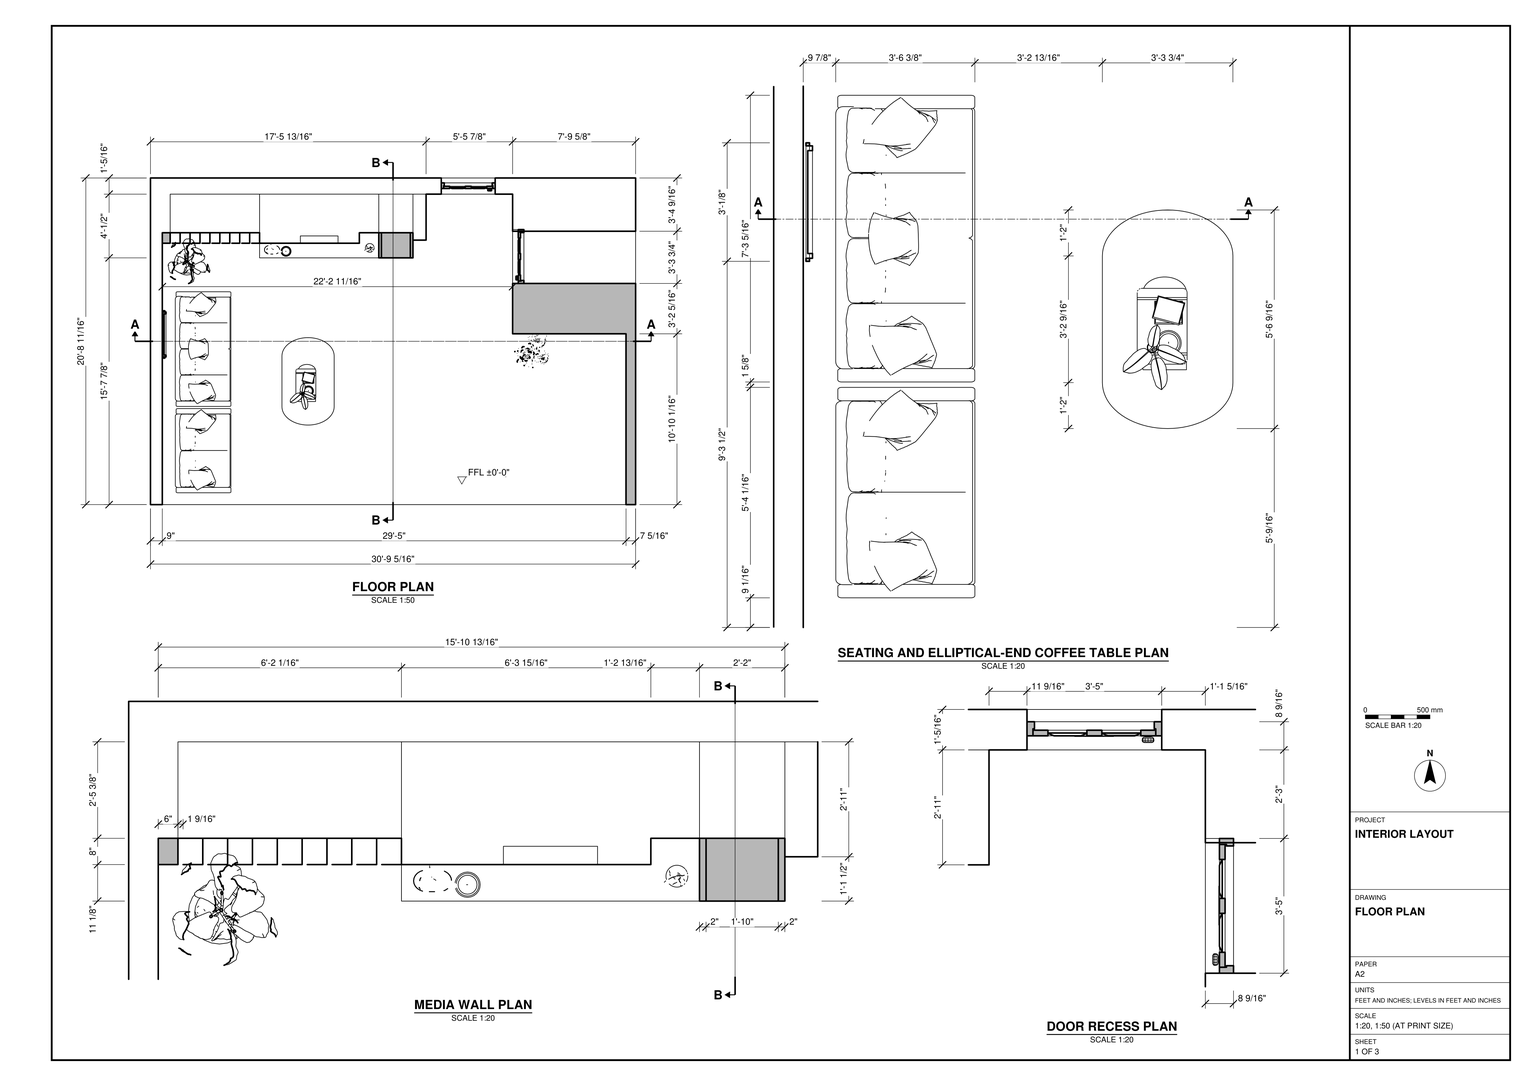
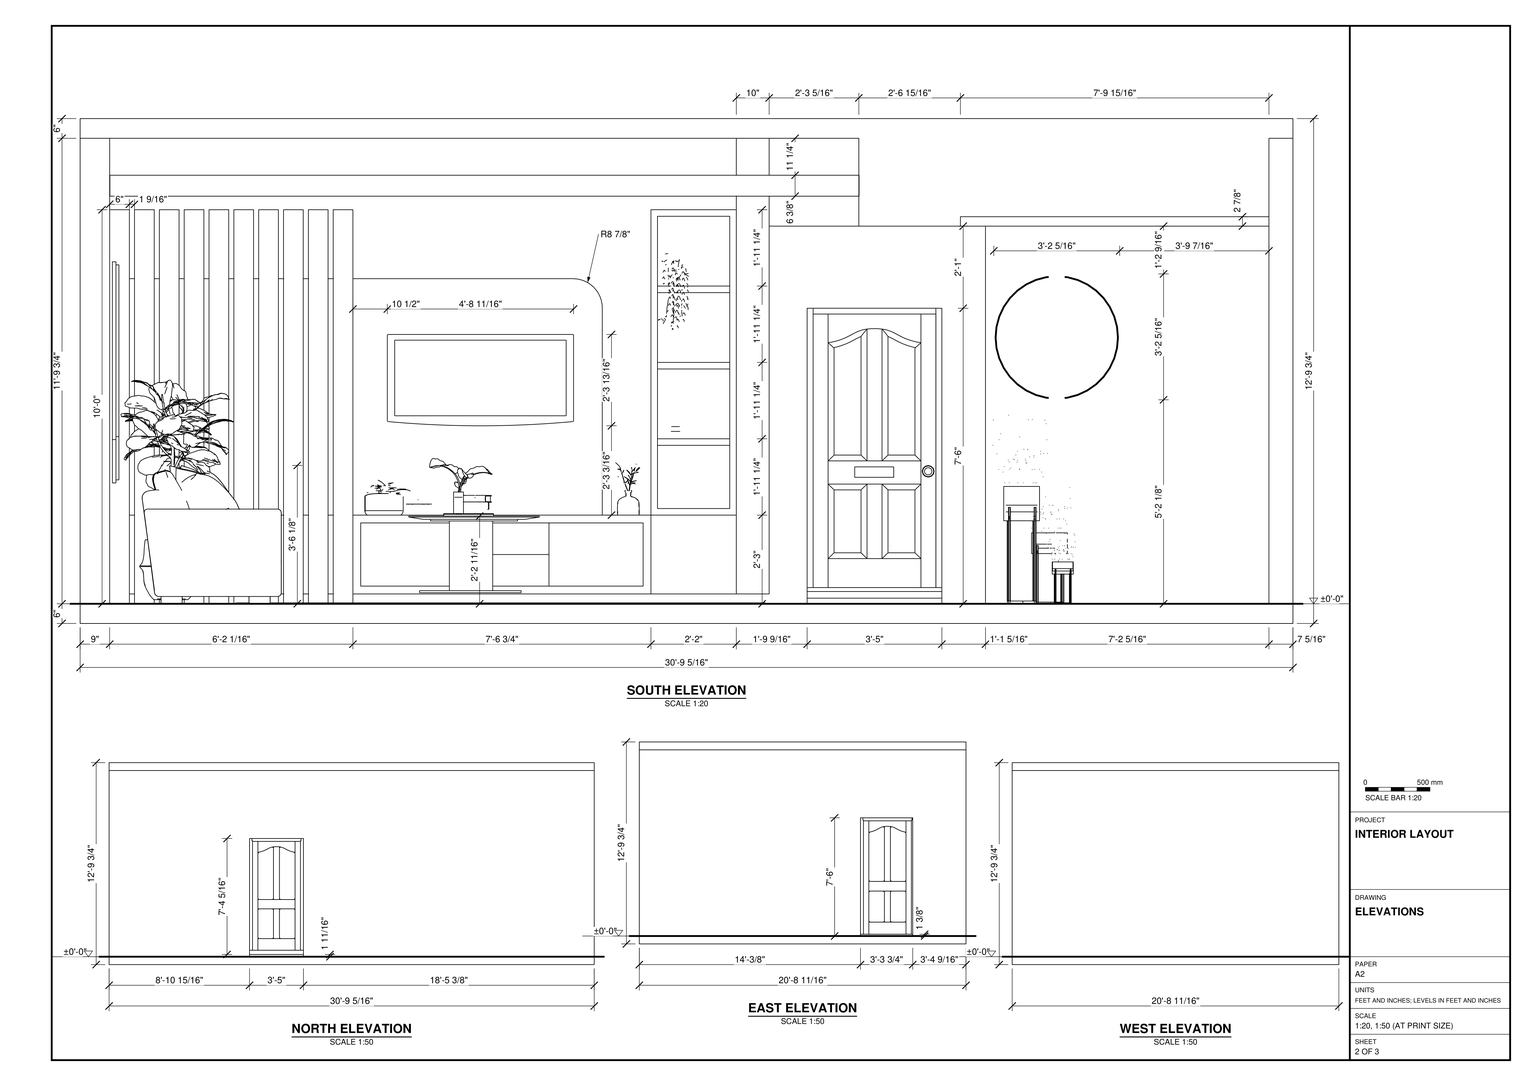
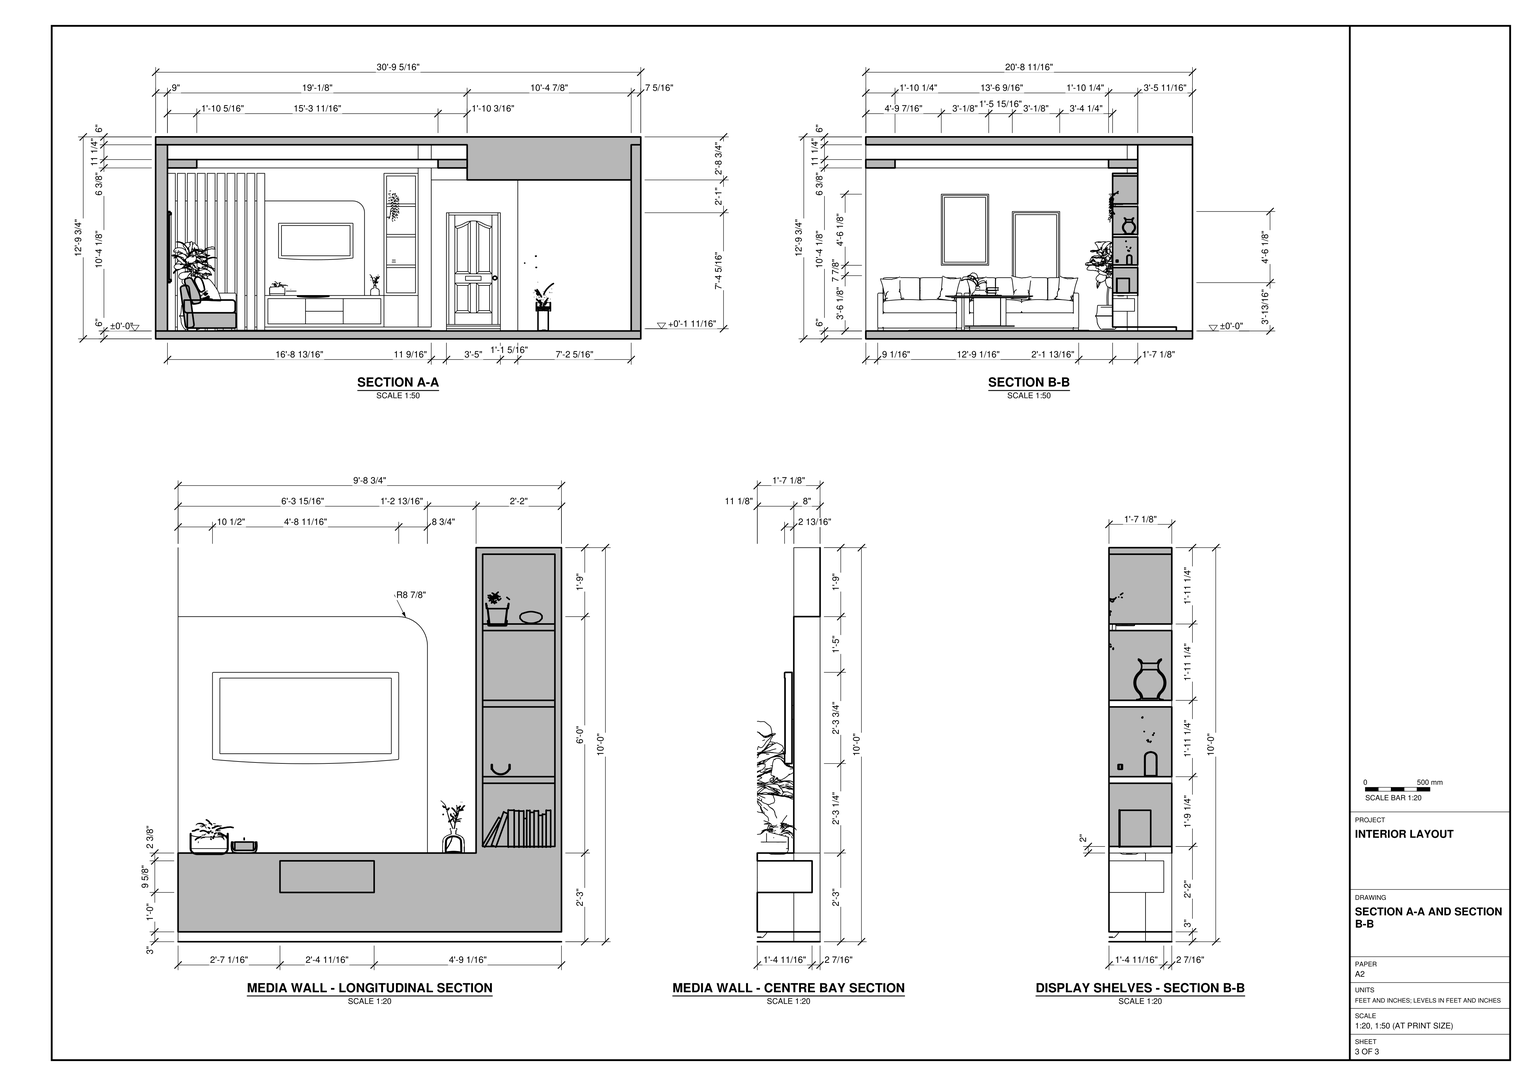
Build the living room in SketchUp from task_files/diagram_01.pdf. Work in feet and inches. Set the finished floor at ±0'-0" and make the overall model 30'-9 5/16" wide, 20'-8 11/16" deep and 12'-9 3/4" high. Use the floor plan to lay out the walls at their drawn thicknesses, including the 9" wall beside the sofas and the 7 5/16" wall opposite. Form the stepped recess with a panelled door in each of its perpendicular walls. Use the sections to set the floor and roof slab thicknesses and the changes in ceiling height.

Build the media wall in the order shown in the south elevation: vertical slats at the sofa end, a low storage cabinet beneath the screen, and a tall open display unit beside the door recess. Follow the joinery sections for the cabinet fronts, shelf depths and rounded upper corner of the screen backing. Place the sofas end to end along the side wall, with the elliptical-end coffee table in front of them. Use the enlarged furniture plan for their sizes, spacing and orientation. Decor and loose items, including the cushions, plants, books and wall clock, may be any suitable library components placed as shown.

Keep the walls, slabs and other shell elements separate as groups or components. Make each furniture or joinery piece a separate group or component and use components for repeated parts. Save one SketchUp model as output_files/living_room_and_its_built_in_media_wall.skp.

# SketchUp Ruby script. Lengths in inches.
U = 1.inch
M = Sketchup.active_model
def pt(a) = Geom::Point3d.new(a.map { |v| v * U })
def face(e, loops, mat)
  f = e.add_face(loops[0].map { |a| pt(a) })
  loops[1..].each { |l| e.add_face(l.map { |a| pt(a) }).erase! }
  f.material = f.back_material = mat if mat
  f
end
# faces: each face lists its corners as indices into pts; further lists are holes
def faces(e, pts, list, mat = nil) = list.each { |f| face(e, (f[0].is_a?(Array) ? f : [f]).map { |l| l.map { |i| pts[i] } }, mat) }
# xy, xz, yz: faces in a plane at the given z, y or x. An outline is a flat list of corners, or four numbers for a rectangle; further outlines are holes
def ring(l) = l.size == 4 ? [[l[0], l[1]], [l[2], l[1]], [l[2], l[3]], [l[0], l[3]]] : l.each_slice(2).to_a
def flat(e, list, mat, &to3) = list.each { |f| face(e, (f[0].is_a?(Array) ? f : [f]).map { |l| ring(l).map { |u, v| to3.(u, v) } }, mat) }
def xy(e, z, list, mat = nil) = flat(e, list, mat) { |x, y| [x, y, z] }
def xz(e, y, list, mat = nil) = flat(e, list, mat) { |x, z| [x, y, z] }
def yz(e, x, list, mat = nil) = flat(e, list, mat) { |y, z| [x, y, z] }
def lines(e, pts, list) = list.each { |a, b| e.add_line(pt(pts[a]), pt(pts[b])) }
# prism: a flat outline (further loops are holes) pulled along v
def prism(e, loops, v, mat = nil)
  f = face(e, loops, mat); d = Geom::Vector3d.new(v.map { |x| x * U })
  f.pushpull(f.normal.samedirection?(d) ? d.length : -d.length)
end
def box(e, o, s, mat = nil) = prism(e, [[o, [o[0] + s[0], o[1], o[2]], [o[0] + s[0], o[1] + s[1], o[2]], [o[0], o[1] + s[1], o[2]]]], [0, 0, s[2]], mat)
def at(x, y, z, deg = 0) = Geom::Transformation.translation(pt([x, y, z])) * Geom::Transformation.rotation(ORIGIN, Z_AXIS, deg.degrees)
def axes(o, x, y, z) = Geom::Transformation.new([*x, 0, *y, 0, *z, 0, *pt(o).to_a, 1])
def part(name) = M.definitions.add(name)
# library, detail: a bought-in or finely detailed component or shape, given as its bounding box
def library(name, o, s) = part(name).tap { |d| box(d.entities, o, s) }
def detail(e, o, s) = box(e.add_group.entities, o, s)
def put(e, d, t, mat = nil) = e.add_instance(d, t).tap { |i| i.material = mat if mat }
def group(e, t, mat = nil) = e.add_group.tap { |g| g.transformation = t; g.material = mat if mat }.entities
root = M.entities
M.materials.add("Material~69").color = [153, 142, 126]
M.materials.add("[Color C02]").color = [255, 204, 153]
M.materials.add("[Color C06]").color = [234, 148, 63]
M.materials.add("[Color C08]").color = [102, 51, 0]
M.materials.add("[Color E01]").color = [255, 255, 204]
M.materials.add("[Color M07]").color = [58, 58, 58]
M.materials.add("[Translucent Glass Gray]").color = [128, 128, 128]
M.materials["[Translucent Glass Gray]"].alpha = 0.5
c1 = library("door2",[0,0,0],[35.42,7.875,78.74])
c2 = library("Plant+Philodendron+Scandens",[-5.75,-7.35,0],[25.95,25.95,24.43])
c3 = library("stone+Jar+4",[7.875,-15.36,0],[26.34,31.07,40.68])
c4 = library("Plant+2 (1)",[-9.13,-9.52,0],[51.76,51.77,66.88])
c5 = library("Plant1",[-0.09,-1.87,0],[3.22,5.78,8.62])
c6 = library("Candle Holder",[-3.9375,-3.9375,0],[7.875,7.875,5.91])
c7 = library("60974+Wall+Clock+Clip+107cm",[-21.0625,-2.75,0],[42.125,5.01,42.125])
c8 = library("Group145\#2",[5.875,6.46,9.56],[20.8,10.13,11.36])
c9 = library("Untitled (9)",[-0.59,0,0],[15.67,17.07,16.5])
c10 = library("Untitled\#1",[82.71,28.87,-11.8125],[39.77,1.97,25.2])
c11 = library("plants",[-0.26,-0.03,0],[11.57,13.37,22.79])
c12 = part("Group\#1")
xz(c12.entities,0,[[0,0,6,120]])
yz(c12.entities,6,[[0,0,8,120]])
c13 = library("Upholstered sofa \#1",[0.125,0,0],[94.22,38.9,37.51])
c14 = library("Upholstered sofa",[0.125,0,0],[128.54,38.9,37.5625])
c15 = part("3DGeom~69_Defintion")
xy(c15.entities,14.55,[[-498.55,-461.83,498.98,-461.4,-498.98,461.4],[498.98,-461.4,498.55,461.83,-498.98,461.4]],"Material~69")
p = [[-498.55,-461.83,14.55],[-500,-461.99,12.51],[499.14,-462.85,12.51],[498.98,-462.58,13.6875],[498.98,-461.4,14.55],[500,461.99,12.51],
  [-498.98,461.4,14.55],[-499.14,462.85,12.51],[-499.73,-461.83,13.6875],[499.73,461.83,13.6875],[-498.98,462.58,13.6875],[498.55,461.83,14.55]]
faces(c15.entities,p,[[0,1,2],[2,3,0],[4,2,5],[2,4,3],[6,7,1],[1,8,6],[1,0,8],[5,9,4],
  [7,6,10],[11,5,7],[7,10,11],[5,11,9],[3,4,0],[8,0,6],[9,11,4],[10,6,11]],"Material~69")
c16 = part("Group209\#1")
put(c16.entities,c15,axes([-3.37,-15.69,-1.69],[0,-0.13066,0],[0.16609,0,0],[0,0,0.13066]),"Material~69")
c17 = part("Group208\#1")
put(c17.entities,c16,at(0,0,0))
c18 = library("Group\#4",[0,0,0],[84.25,35.43,29.53])
c19 = library("Group\#7",[-0.77,-0.05,0],[14.94,14.79,13.98])
c20 = library("Group\#8",[-6.09,-4.97,0],[28.53,35.82,18.15])
c21 = library("Group\#30",[0,0,0],[159.9,159.9,209.38])
xy(root,-6,[[0,0,369.3125,248.6875]])
xy(root,0,[[0,0,9,0,9,207,15,207,15,236.375,221.375,236.375,221.375,248.6875,0,248.6875],[9,0,362,0,362,130.0625,275.6875,130.0625,275.6875,168.375,369.3125,168.375,369.3125,208.125,275.6875,208.125,275.6875,236.375,262.41,236.375,262.41,248.6875,221.375,248.6875,221.375,236.375,15,236.375,15,199,9,199],[362,0,369.3125,0,369.3125,168.375,275.6875,168.375,275.6875,130.0625,362,130.0625],[9,199,15,207],[275.6875,208.125,369.3125,208.125,369.3125,248.6875,262.41,248.6875,262.41,236.375,275.6875,236.375]])
xy(root,3,[[83.0625,187.875,173.8125,236.375],[173.8125,187.875,199.8125,236.375],[199.8125,201.375,209.8125,236.375],[15,207,83.0625,236.375]])
xy(root,15,[[114.1,187.875,142.77,204.5625]],"[Color M07]")
xy(root,24.62,[[114.1,187.875,142.77,204.5625]])
xy(root,27,[[83.0625,187.875,173.8125,187.875,173.8125,207,159,207,159,199,83.0625,199]],"[Color C06]")
xy(root,29,[[175.8125,187.875,197.8125,207]])
xy(root,48.25,[[175.8125,187.875,197.8125,207]])
xy(root,50.25,[[175.8125,187.875,197.8125,207]])
xy(root,71.5,[[175.8125,187.875,197.8125,207]])
xy(root,73.5,[[175.8125,187.875,197.8125,207]])
xy(root,90,[[275.6875,168.375,369.3125,208.125],[221.375,236.375,262.41,248.6875]])
xy(root,94.75,[[175.8125,187.875,197.8125,207]])
xy(root,96.75,[[175.8125,187.875,197.8125,207]])
xy(root,99,[[83.0625,199,150.1,207]])
xy(root,115,[[237.125,0,237.125,201.375,209.8125,201.375,209.8125,236.375,275.6875,236.375,275.6875,130.0625,362,130.0625,362,96.66,268.05,96.66,268.05,0]],"[Color E01]")
xy(root,117.875,[[268.05,0,362,96.66]],"[Color E01]")
xy(root,118,[[175.8125,187.875,197.8125,207]])
xy(root,120,[[173.8125,187.875,199.8125,207],[9,199,15,207],[16.5625,199,22.5625,207],[24.125,199,30.125,207],[31.6875,199,37.6875,207],
  [39.25,199,45.25,207],[46.8125,199,52.8125,207],[54.375,199,60.375,207],[61.9375,199,67.9375,207],[69.5,199,75.5,207],
  [77.0625,199,83.0625,207]])
xy(root,124.12,[[[9.08,0,9.08,207,199.89,207,199.89,201.375,237.2,201.375,237.2,0],[31.31,22.23,214.97,184.77]]],"[Color E01]")
xy(root,130.5,[[[9.08,0,237.2,0,237.2,201.375,199.89,201.375,199.89,207,9.08,207],[31.31,22.23,214.97,184.77]]])
xy(root,130.5,[[31.31,22.23,214.97,184.77]],"[Color E01]")
xy(root,141.75,[[0,0,0,248.6875,369.3125,248.6875,369.3125,0,362,0,362,130.0625,275.6875,130.0625,275.6875,236.375,209.8125,236.375,209.8125,201.375,199.8125,201.375,199.8125,207,9,207,9,0],[9,0,9,207,199.8125,207,199.8125,201.375,237.125,201.375,237.125,0]])
xy(root,147.75,[[0,0,369.3125,248.6875]])
xz(root,0,[[0,-6,369.3125,0],[0,0,9,141.75],[362,0,369.3125,141.75],[9.08,124.12,237.125,130.5],[237.125,124.12,237.2,130.5]])
xz(root,0,[[237.125,115,268.05,115,268.05,117.875,362,117.875,362,141.75,369.3125,141.75,369.3125,147.75,0,147.75,0,141.75,237.125,141.75,237.125,130.5,237.2,130.5,237.2,124.12,237.125,124.12]],"[Color C02]")
xz(root,22.23,[[31.31,124.12,214.97,130.5]])
xz(root,96.66,[[268.05,115,362,117.875]])
xz(root,130.0625,[[275.6875,115,362,141.75]])
xz(root,130.0625,[[275.6875,0,362,115]],"[Color C02]")
xz(root,168.375,[[275.6875,0,369.3125,90]])
xz(root,184.77,[[31.31,124.12,214.97,130.5]],"[Color E01]")
xz(root,187.875,[[85.44,5.38,114.1,24.62],[114.1,5.38,142.77,15],[142.77,5.38,171.44,24.62]])
xz(root,187.875,[[[83.0625,3,173.8125,27],[85.44,5.38,171.44,24.62]],[173.8125,3,199.8125,27],[[173.8125,27,199.8125,120],[175.8125,29,197.8125,118]],[175.8125,48.25,197.8125,50.25],[175.8125,71.5,197.8125,73.5],
  [175.8125,94.75,197.8125,96.75]],"[Color C06]")
xz(root,187.875,[[175.8125,29,197.8125,48.25],[175.8125,50.25,197.8125,71.5],[175.8125,73.5,197.8125,94.75],[175.8125,96.75,197.8125,118]],"[Translucent Glass Gray]")
xz(root,199,[[83.0625,27,159,27,159,90.1,158.92,91.26,158.7,92.4,158.32,93.51,157.81,94.55,157.16,95.52,156.39,96.39,155.52,97.16,154.55,97.81,153.51,98.32,152.4,98.7,151.26,98.92,150.1,99,83.0625,99]],"[Color C02]")
xz(root,201.375,[[199.89,124.12,209.8125,130.5],[209.8125,124.12,209.89,130.5],[209.89,124.12,237.125,130.5],[237.125,124.12,237.2,130.5],[209.8125,130.5,237.125,141.75]])
xz(root,201.375,[[199.8125,3,209.8125,3,209.8125,124.12,199.89,124.12,199.89,130.5,209.8125,130.5,209.8125,141.75,199.8125,141.75],[209.8125,115,237.125,124.12]],"[Color C02]")
xz(root,204.5625,[[114.1,15,142.77,24.62]],"[Color M07]")
xz(root,207,[[9,0,15,120],[15,3,83.0625,27],[15,27,83.0625,99],[[173.8125,27,199.8125,120],[175.8125,29,197.8125,118]],[175.8125,29,197.8125,48.25],
  [175.8125,50.25,197.8125,71.5],[175.8125,73.5,197.8125,94.75],[175.8125,96.75,197.8125,118],[9.08,124.12,199.8125,130.5],[199.8125,124.12,199.89,130.5]])
xz(root,207,[[159,27,173.8125,27,173.8125,120,199.8125,120,199.8125,124.12,9.08,124.12,9.08,130.5,199.8125,130.5,199.8125,141.75,9,141.75,9,120,15,120,15,99,150.1,99,151.26,98.92,152.4,98.7,153.51,98.32,154.55,97.81,155.52,97.16,156.39,96.39,157.16,95.52,157.81,94.55,158.32,93.51,158.7,92.4,158.92,91.26,159,90.1]],"[Color C02]")
xz(root,208.125,[[275.6875,0,369.3125,90]],"[Color C02]")
xz(root,236.375,[[209.8125,115,275.6875,141.75]])
xz(root,236.375,[[15,0,221.375,0,221.375,90,262.41,90,262.41,0,275.6875,0,275.6875,115,209.8125,115,209.8125,3,15,3]],"[Color C02]")
xz(root,248.6875,[[0,-6,369.3125,0],[0,0,0,141.75,369.3125,141.75,369.3125,0,262.41,0,262.41,90,221.375,90,221.375,0],[0,141.75,369.3125,147.75]])
yz(root,0,[[0,-6,248.6875,0],[0,0,248.6875,141.75],[0,141.75,248.6875,147.75]])
yz(root,9,[[199,0,207,120],[199,120,207,141.75]])
yz(root,9,[[0,0,199,141.75]],"[Color C02]")
yz(root,9.08,[[0,124.12,199,130.5],[199,124.12,207,130.5]])
yz(root,15,[[207,0,236.375,3]])
yz(root,31.31,[[22.23,124.12,184.77,130.5]],"[Color E01]")
yz(root,83.0625,[[187.875,3,207,27],[199,27,207,99]])
yz(root,114.1,[[187.875,15,204.5625,24.62]],"[Color M07]")
yz(root,142.77,[[187.875,15,204.5625,24.62]],"[Color M07]")
yz(root,159,[[199,27,207,90.1]])
yz(root,173.8125,[[187.875,27,207,120]],"[Color C06]")
yz(root,175.8125,[[187.875,29,207,48.25],[187.875,48.25,207,50.25],[187.875,50.25,207,71.5],[187.875,71.5,207,73.5],[187.875,73.5,207,94.75],
  [187.875,94.75,207,96.75],[187.875,96.75,207,118]])
yz(root,197.8125,[[187.875,29,207,48.25],[187.875,48.25,207,50.25],[187.875,50.25,207,71.5],[187.875,71.5,207,73.5],[187.875,73.5,207,94.75],
  [187.875,94.75,207,96.75],[187.875,96.75,207,118]])
yz(root,199.8125,[[201.375,27,207,120],[201.375,120,207,141.75]])
yz(root,199.8125,[[187.875,3,201.375,120]],"[Color C06]")
yz(root,199.89,[[201.375,124.12,207,130.5]])
yz(root,209.8125,[[201.375,3,236.375,115],[201.375,115,236.375,141.75]])
yz(root,214.97,[[22.23,124.12,184.77,130.5]],"[Color E01]")
yz(root,221.375,[[236.375,0,248.6875,90]])
yz(root,237.125,[[0,115,201.375,141.75]],"[Color E01]")
yz(root,237.2,[[0,124.12,5.4375,130.5],[5.4375,124.12,201.375,130.5]])
yz(root,262.41,[[236.375,0,248.6875,90]])
yz(root,268.05,[[0,115,96.66,117.875]])
yz(root,275.6875,[[130.0625,115,236.375,141.75]])
yz(root,275.6875,[[130.0625,0,130.0625,115,236.375,115,236.375,0,208.125,0,208.125,90,168.375,90,168.375,0]],"[Color C02]")
yz(root,362,[[0,0,0,117.875,96.66,117.875,96.66,115,130.0625,115,130.0625,0],[96.66,115,96.66,117.875,0,117.875,0,141.75,130.0625,141.75,130.0625,115]])
yz(root,369.3125,[[0,-6,248.6875,0],[0,0,168.375,0,168.375,90,208.125,90,208.125,0,248.6875,0,248.6875,141.75,0,141.75],[0,141.75,248.6875,147.75]])
p = [[159,207,90.1],[158.92,207,91.26],[158.92,199,91.26],[159,199,90.1],[158.7,207,92.4],[158.7,199,92.4],
  [158.32,207,93.51],[158.32,199,93.51],[157.81,207,94.55],[157.81,199,94.55],[157.16,207,95.52],[157.16,199,95.52],
  [156.39,207,96.39],[156.39,199,96.39],[155.52,207,97.16],[155.52,199,97.16],[154.55,207,97.81],[154.55,199,97.81],
  [153.51,207,98.32],[153.51,199,98.32],[152.4,207,98.7],[152.4,199,98.7],[151.26,207,98.92],[151.26,199,98.92],
  [150.1,207,99],[150.1,199,99]]
faces(root,p,[[0,1,2,3],[1,4,5,2],[4,6,7,5],[6,8,9,7],[8,10,11,9],[10,12,13,11],[12,14,15,13],[14,16,17,15],
  [16,18,19,17],[18,20,21,19],[20,22,23,21],[22,24,25,23]])
put(root,c1,axes([221.375,236.375,1.71],[1.1584,0,0],[0,1.09,0],[0,0,1.1213]))
put(root,c1,axes([275.6875,209.41,-1.97],[0,-1.1584,0],[1.09,0,0],[0,0,1.16802]))
put(root,c2,at(173.16,184.4375,82.79))
put(root,c3,axes([185,200.19,74.86],[0.3096,0,0],[0,0.3096,0],[0,0,0.3096]))
put(root,c4,at(12.39,167.17,1.26))
put(root,c5,axes([163.09,198.79,27],[0,-2.19,0],[2.19,0,0],[0,0,2.19]))
put(root,c6,at(103.18,192.875,27))
put(root,c7,axes([297.39,119.2,62.12],[0.91,0,0],[0,0.91,0],[0,0,0.91]))
put(root,c8,at(169.85,184.375,19.23))
put(root,c9,axes([177.88,187.875,50.25],[1.11,0,0],[0,1.11,0],[0,0,1.11]))
put(root,c3,axes([176.64,200.28,73.5],[0.3096,0,0],[0,0.3096,0],[0,0,0.3096]))
put(root,c10,axes([-24.4,155.03,67.24],[1.426,0,0],[0,1.426,0],[0,0,1.10372]))
put(root,c11,axes([274.14,101.68,0],[2.69,0,0],[0,2.69,0],[0,0,2.69]))
put(root,c12,at(9,199,0),"[Color C08]")
put(root,c12,at(16.5625,199,0),"[Color C08]")
put(root,c12,at(24.125,199,0),"[Color C08]")
put(root,c12,at(31.6875,199,0),"[Color C08]")
put(root,c12,at(39.25,199,0),"[Color C08]")
put(root,c12,at(46.8125,199,0),"[Color C08]")
put(root,c12,at(54.375,199,0),"[Color C08]")
put(root,c12,at(61.9375,199,0),"[Color C08]")
put(root,c12,at(69.5,199,0),"[Color C08]")
put(root,c12,at(77.0625,199,0),"[Color C08]")
g1 = group(root,at(9.83,57.45,50))
xy(g1,0,[[0,0,1.08,36.1]])
xy(g1,0.9375,[[0,0.9375,1.08,35.16],[1.08,0.9375,1.99,35.16]])
xy(g1,2.38,[[0.54,2.38,1.99,33.72]])
xy(g1,51.76,[[0.54,2.38,1.99,33.72]])
xy(g1,53.21,[[0,0.9375,1.08,35.16],[1.08,0.9375,1.99,35.16]])
xy(g1,54.14,[[0,0,1.08,36.1]])
xz(g1,0,[[0,0,1.08,54.14]])
xz(g1,0.9375,[[0,0.9375,1.08,53.21],[1.08,0.9375,1.99,53.21]])
xz(g1,2.38,[[0.54,2.38,1.99,51.76]])
xz(g1,33.72,[[0.54,2.38,1.99,51.76]])
xz(g1,35.16,[[0,0.9375,1.08,53.21],[1.08,0.9375,1.99,53.21]])
xz(g1,36.1,[[0,0,1.08,54.14]])
yz(g1,0,[[[0,0,36.1,54.14],[0.9375,0.9375,35.16,53.21]]])
yz(g1,0.54,[[2.38,2.38,33.72,51.76]])
yz(g1,1.08,[[[0,0,36.1,54.14],[0.9375,0.9375,35.16,53.21]]])
yz(g1,1.99,[[[0.9375,0.9375,35.16,53.21],[2.38,2.38,33.72,51.76]]])
g2 = group(root,at(9.83,111.5,36.8))
xy(g2,0,[[0,0,1.08,36.1]])
xy(g2,0.9375,[[0,0.9375,1.08,35.16],[1.08,0.9375,1.99,35.16]])
xy(g2,2.38,[[0.54,2.38,1.99,33.72]])
xy(g2,51.76,[[0.54,2.38,1.99,33.72]])
xy(g2,53.21,[[0,0.9375,1.08,35.16],[1.08,0.9375,1.99,35.16]])
xy(g2,54.14,[[0,0,1.08,36.1]])
xz(g2,0,[[0,0,1.08,54.14]])
xz(g2,0.9375,[[0,0.9375,1.08,53.21],[1.08,0.9375,1.99,53.21]])
xz(g2,2.38,[[0.54,2.38,1.99,51.76]])
xz(g2,33.72,[[0.54,2.38,1.99,51.76]])
xz(g2,35.16,[[0,0.9375,1.08,53.21],[1.08,0.9375,1.99,53.21]])
xz(g2,36.1,[[0,0,1.08,54.14]])
yz(g2,0,[[[0,0,36.1,54.14],[0.9375,0.9375,35.16,53.21]]])
yz(g2,0.54,[[2.38,2.38,33.72,51.76]])
yz(g2,1.08,[[[0,0,36.1,54.14],[0.9375,0.9375,35.16,53.21]]])
yz(g2,1.99,[[[0.9375,0.9375,35.16,53.21],[2.38,2.38,33.72,51.76]]])
g3 = group(root,at(61.26,9.04,0.03))
put(g3,c13,axes([0,-0.09,0],[0,0.68172,0],[-1.10207,0,0],[0,0,1.13261]))
put(g3,c14,axes([-0.03,65.64,0],[0,0.68172,0],[-1.10207,0,0],[0,0,1.13261]))
put(root,c17,axes([131.61,117.69,0.06],[1.05,0,0],[0,1.05,0],[0,0,1.05]))
put(root,c18,axes([100.08,127.15,3.38],[0,-0.79,0],[1.1218,0,0],[0,0,0.79]))
put(root,c19,axes([86.69,199.77,26.62],[0,-0.84,0],[1,0,0],[0,0,0.87]))
put(root,c20,at(106.42,72.41,26.71))
put(root,c21,axes([186.8125,187.875,96.75],[0.04664,0,0],[0,0.04664,0],[0,0,0.04664]))
